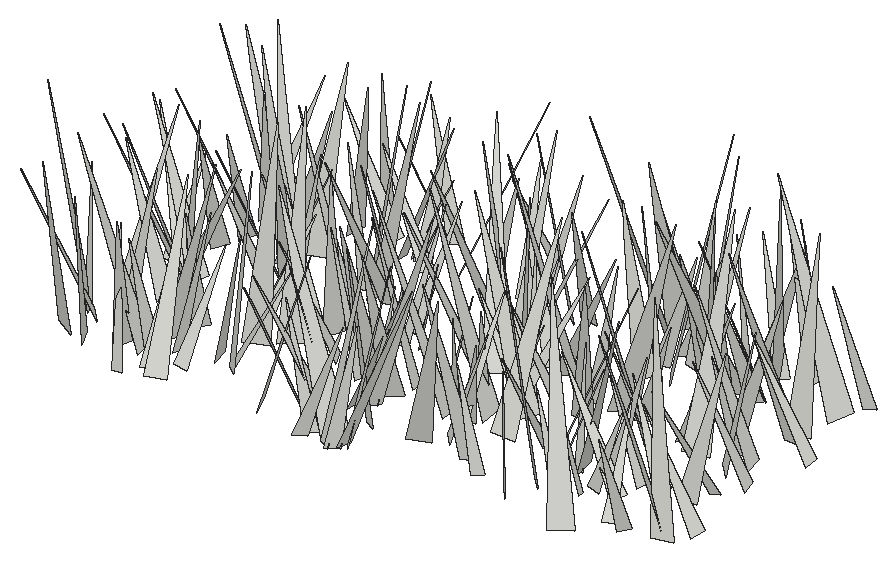
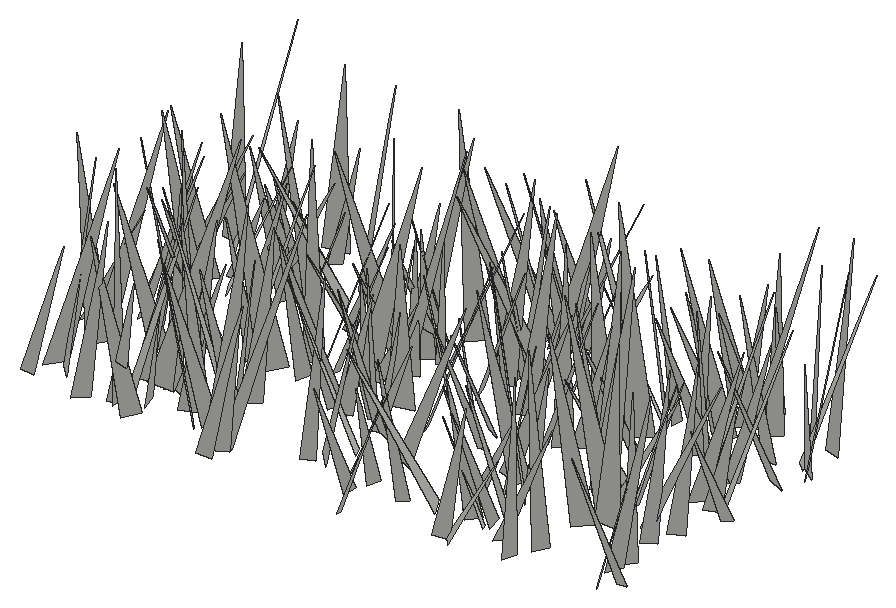
# SketchUp Ruby script. Lengths in inches.
U = 1.inch
M = Sketchup.active_model
def pt(a) = Geom::Point3d.new(a.map { |v| v * U })
def face(e, loops, mat)
  f = e.add_face(loops[0].map { |a| pt(a) })
  loops[1..].each { |l| e.add_face(l.map { |a| pt(a) }).erase! }
  f.material = f.back_material = mat if mat
  f
end
# faces: each face lists its corners as indices into pts; further lists are holes
def faces(e, pts, list, mat = nil) = list.each { |f| face(e, (f[0].is_a?(Array) ? f : [f]).map { |l| l.map { |i| pts[i] } }, mat) }
# xy, xz, yz: faces in a plane at the given z, y or x. An outline is a flat list of corners, or four numbers for a rectangle; further outlines are holes
def ring(l) = l.size == 4 ? [[l[0], l[1]], [l[2], l[1]], [l[2], l[3]], [l[0], l[3]]] : l.each_slice(2).to_a
def flat(e, list, mat, &to3) = list.each { |f| face(e, (f[0].is_a?(Array) ? f : [f]).map { |l| ring(l).map { |u, v| to3.(u, v) } }, mat) }
def xy(e, z, list, mat = nil) = flat(e, list, mat) { |x, y| [x, y, z] }
def xz(e, y, list, mat = nil) = flat(e, list, mat) { |x, z| [x, y, z] }
def yz(e, x, list, mat = nil) = flat(e, list, mat) { |y, z| [x, y, z] }
def lines(e, pts, list) = list.each { |a, b| e.add_line(pt(pts[a]), pt(pts[b])) }
# prism: a flat outline (further loops are holes) pulled along v
def prism(e, loops, v, mat = nil)
  f = face(e, loops, mat); d = Geom::Vector3d.new(v.map { |x| x * U })
  f.pushpull(f.normal.samedirection?(d) ? d.length : -d.length)
end
def box(e, o, s, mat = nil) = prism(e, [[o, [o[0] + s[0], o[1], o[2]], [o[0] + s[0], o[1] + s[1], o[2]], [o[0], o[1] + s[1], o[2]]]], [0, 0, s[2]], mat)
def at(x, y, z, deg = 0) = Geom::Transformation.translation(pt([x, y, z])) * Geom::Transformation.rotation(ORIGIN, Z_AXIS, deg.degrees)
def axes(o, x, y, z) = Geom::Transformation.new([*x, 0, *y, 0, *z, 0, *pt(o).to_a, 1])
def part(name) = M.definitions.add(name)
# library, detail: a bought-in or finely detailed component or shape, given as its bounding box
def library(name, o, s) = part(name).tap { |d| box(d.entities, o, s) }
def detail(e, o, s) = box(e.add_group.entities, o, s)
def put(e, d, t, mat = nil) = e.add_instance(d, t).tap { |i| i.material = mat if mat }
def group(e, t, mat = nil) = e.add_group.tap { |g| g.transformation = t; g.material = mat if mat }.entities
root = M.entities
c1 = part("fur_instance\#9")
p = [[0.8125,0,1.79],[0.67,-0.02,1.48],[0,-0.11,0],[0,0.11,0]]
faces(c1.entities,p,[[0,1,2,3]])
put(root,c1,axes([454.98,138.05,-21.66],[-2.48382,-6.27006,1.58629],[-6.2632,2.75568,1.08533],[1.61318,1.04494,6.65621]))
put(root,c1,axes([476.97,136.47,-21.66],[3.46953,-2.67132,1.40146],[-2.94376,-3.4648,0.68347],[-0.65905,1.41311,4.3251]))
put(root,c1,axes([474.43,136.51,-21.66],[3.70527,-2.55389,0.75103],[-2.66189,-3.54115,1.0909],[0.02774,1.32414,4.36593]))
put(root,c1,axes([456.74,137.75,-21.66],[4.97052,1.68586,2.30908],[2.28367,-5.12743,-1.17229],[-1.72012,-1.9358,5.11604]))
put(root,c1,axes([460.83,135.75,-21.66],[0.97276,4.45119,0.9772],[4.35496,-1.20232,1.14148],[-1.3425,-0.67498,4.41093]))
put(root,c1,axes([459.04,138.55,-21.66],[4.90376,-2.85552,0.72078],[-2.73926,-4.93651,-0.92072],[-1.08166,-0.44414,5.59939]))
put(root,c1,axes([475.1,138.93,-21.66],[-5.50457,-1.9976,0.13924],[-1.94432,5.42927,1.02602],[0.47897,-0.91798,5.76524]))
put(root,c1,axes([474.72,137.23,-21.66],[0.57769,-3.84784,2.16026],[-4.16363,-1.197,-1.01866],[-1.46176,1.88882,3.75525]))
put(root,c1,axes([461.22,138.875,-21.66],[3.60801,-2.69307,1.35493],[-2.4926,-3.85347,-1.02171],[-1.69571,-0.06573,4.3848]))
put(root,c1,axes([470.25,137.9,-21.66],[6.04949,2.12455,0.78775],[2.22415,-5.99674,-0.90711],[-0.43293,-1.1207,6.34722]))
put(root,c1,axes([455.41,140.42,-21.66],[-4.43936,-4.76816,0.23664],[-4.66276,4.39992,1.18262],[1.02469,-0.63608,6.40661]))
put(root,c1,axes([488.52,138.7,-21.66],[3.47548,2.68418,2.07766],[3.24177,-3.50628,-0.89294],[-1.00618,-2.02524,4.29959]))
put(root,c1,axes([460.34,139.04,-21.66],[-7.46338,-1.41905,1.28497],[-1.31215,7.55774,0.72509],[1.39396,-0.48353,7.56241]))
put(root,c1,axes([475.88,138.03,-21.66],[-6.89397,4.20656,1.53795],[4.42912,6.82252,1.19307],[0.66584,-1.82904,7.9874]))
put(root,c1,axes([477.26,137.21,-21.66],[6.02676,-0.13267,0.65935],[-0.25057,-5.95995,1.09109],[-0.62414,1.1116,5.92866]))
put(root,c1,axes([474.29,139.79,-21.66],[-3.67064,-4.64361,1.03864],[-4.58105,3.8034,0.81465],[1.28682,0.29416,5.86285]))
put(root,c1,axes([497.07,139.62,-21.66],[2.57242,-3.23839,0.522],[-3.12857,-2.6216,-0.84629],[-0.98573,-0.13048,4.04824]))
put(root,c1,axes([493.08,138.49,-21.66],[-3.28307,2.60382,1.30489],[2.8552,3.26547,0.66758],[0.57484,-1.34832,4.13676]))
put(root,c1,axes([462.01,137.22,-21.66],[-2.71251,3.20119,0.88639],[3.03008,2.85354,-1.03292],[1.36084,0.02704,4.06674]))
put(root,c1,axes([494.09,137.1875,-21.66],[-3.06885,7.2619,1.47031],[7.40414,2.94663,0.90053],[-0.27521,-1.70206,7.83212]))
put(root,c1,axes([480.46,140.51,-21.66],[3.94338,-5.9757,0.15667],[-5.94055,-3.89659,0.90015],[0.66588,0.62564,7.10275]))
put(root,c1,axes([463.16,136.61,-21.66],[-3.56616,5.34471,0.77163],[5.27091,3.64619,-0.89538],[1.17426,-0.13507,6.36253]))
put(root,c1,axes([472.08,139.48,-21.66],[-2.77092,-3.22119,0.17285],[-3.17409,2.68192,-0.90354],[-0.57541,0.71776,4.15182]))
put(root,c1,axes([476.3,136.5,-21.66],[3.93079,5.90323,1.06815],[5.73682,-4.07234,1.39466],[-1.7544,-0.09002,6.95371]))
put(root,c1,axes([477.33,137.4375,-21.66],[-3.93965,-2.75758,3.63418],[-3.8658,4.56754,-0.72493],[2.42222,2.80458,4.7539]))
put(root,c1,axes([498.85,141.17,-21.66],[-5.87389,-5.06073,1.31002],[-4.91563,6.01764,1.20596],[1.77871,-0.08191,7.65893]))
put(root,c1,axes([485.84,139.46,-21.66],[1.13242,-3.28388,1.61058],[-3.44754,-1.52145,-0.67814],[-1.2216,1.24962,3.40681]))
put(root,c1,axes([484.38,140.55,-21.66],[0.42808,-6.23217,1.75974],[-6.34467,-0.7568,-1.13683],[-1.29687,1.64535,6.14254]))
put(root,c1,axes([463.53,138.55,-21.66],[-0.65991,4.20046,0.70673],[4.09857,0.8209,-1.05196],[1.15975,-0.51096,4.1198]))
put(root,c1,axes([464.65,140.98,-21.66],[5.2345,0.58731,0.96902],[0.7581,-5.21929,-0.93179],[-0.84215,-1.04786,5.18428]))
put(root,c1,axes([476.94,140.09,-21.66],[-3.42512,-4.29344,1.99666],[-4.721,3.28594,-1.03273],[0.36395,2.21827,5.39431]))
put(root,c1,axes([462.21,140.04,-21.66],[4.7492,-0.22527,1.39473],[-0.44396,-4.88167,0.72329],[-1.34124,0.81823,4.6992]))
put(root,c1,axes([489.3,140.8125,-21.66],[-5.53788,-5.2946,2.37412],[-5.70348,5.57065,-0.88067],[1.06751,2.29618,7.61087]))
put(root,c1,axes([454.62,140.9,-21.66],[-6.58446,-3.61184,1.85584],[-3.84727,6.67992,-0.64953],[1.29924,1.4758,7.48189]))
put(root,c1,axes([499.61,140.12,-21.66],[-0.81741,7.52572,2.31704],[7.8363,0.54876,0.98214],[-0.77303,-2.39493,7.506]))
put(root,c1,axes([465.74,141.11,-21.66],[3.62695,2.69385,0.06353],[2.59465,-3.4627,-1.30122],[0.7271,-1.08099,4.32648]))
put(root,c1,axes([460.81,140.86,-21.66],[6.40804,-1.16691,1.44574],[-1.35043,-6.49108,0.74636],[-1.27601,1.00946,6.47052]))
put(root,c1,axes([457.27,141.23,-21.66],[1.6675,5.06938,1.93589],[5.41393,-1.41673,-0.95346],[0.36831,-2.12629,5.25072]))
put(root,c1,axes([495.77,139.76,-21.66],[-2.69846,2.82224,0.09608],[2.72603,2.63813,-0.93001],[0.73688,0.57546,3.79233]))
put(root,c1,axes([500.89,141.99,-21.66],[-4.33776,1.46199,0.55548],[1.55819,4.18055,1.16497],[0.13425,-1.28363,4.42678]))
put(root,c1,axes([466.2,140.21,-21.66],[3.82909,4.88275,1.88302],[4.81565,-4.20088,1.10051],[-2.04855,-0.74856,6.10673]))
put(root,c1,axes([475.77,143.82,-21.66],[3.11864,-5.68803,0.55795],[-5.6529,-3.16353,-0.65398],[-0.84244,0.17118,6.45383]))
put(root,c1,axes([454.52,140.9,-21.66],[1.72426,4.07776,1.35625],[4.04188,-2.03524,0.98061],[-1.4597,-0.81871,4.31736]))
put(root,c1,axes([492.26,141.43,-21.66],[-3.43885,-1.25141,0.28396],[-1.28081,3.29756,-0.97876],[-0.07859,1.01608,3.52615]))
put(root,c1,axes([481.72,141.8,-21.66],[3.27603,2.91205,0.73309],[2.99826,-3.11162,-1.03833],[0.1671,-1.26001,4.25844]))
put(root,c1,axes([461.38,143.34,-21.66],[3.51488,-3.51732,0.75482],[-3.443,-3.59499,-0.71937],[-1.04262,0.01399,4.9202]))
put(root,c1,axes([492.47,142.38,-21.66],[0.8957,-3.44027,0.95903],[-3.38159,-0.49886,1.36875],[1.14894,1.21373,3.28089]))
put(root,c1,axes([494.3,142.52,-21.66],[-4.30239,2.31555,0.00735],[2.25428,4.18495,1.12996],[-0.52922,-0.99839,4.75348]))
put(root,c1,axes([475.25,142.56,-21.66],[1.48907,3.83094,1.46531],[4.09712,-1.31638,-0.722],[0.19182,-1.62223,4.04625]))
put(root,c1,axes([475.52,142.05,-21.66],[6.84778,-1.68967,1.39359],[-1.92956,-6.81846,1.21431],[-1.03628,1.53061,6.94784]))
put(root,c1,axes([490.17,141.42,-21.66],[3.37937,2.22818,0.23171],[2.15143,-3.34494,0.78826],[-0.62436,0.53406,3.97033]))
put(root,c1,axes([490.44,144,-21.66],[6.84395,0.46131,0.76105],[0.6015,-6.74756,-1.31919],[-0.65589,-1.3745,6.73144]))
put(root,c1,axes([481.35,144.16,-21.66],[1.83451,-3.56347,0.05806],[-3.52397,-1.80394,0.62811],[0.53227,0.33851,3.95843]))
put(root,c1,axes([480.33,144.3,-21.66],[-0.97115,-4.17934,0.95629],[-4.09852,1.19278,1.05068],[1.25838,0.65947,4.16006]))
put(root,c1,axes([474.66,141.38,-21.66],[6.67299,1.88656,0.54903],[1.75109,-6.59185,1.3677],[-0.89119,1.17381,6.79833]))
put(root,c1,axes([487.18,144.6,-21.66],[-0.13278,-3.81265,0.23397],[-3.74221,0.08288,-0.77308],[-0.76609,0.25594,3.73581]))
put(root,c1,axes([465.32,143.67,-21.66],[-3.47226,6.33449,3.63746],[6.89094,4.17667,-0.69553],[2.42317,-2.80055,7.19017]))
put(root,c1,axes([492.625,143.8125,-21.66],[4.10289,-2.86128,0.97197],[-3.01034,-4.01302,0.89377],[-0.2636,1.29386,4.92156]))
put(root,c1,axes([472.33,145.94,-21.66],[3.11347,-5.57932,0.56956],[-5.54553,-3.1599,-0.63956],[-0.83685,0.18197,6.35716]))
put(root,c1,axes([470.2,145.46,-21.66],[-4.41173,-1.92667,0.46008],[-1.77307,4.34177,1.17998],[0.88316,-0.90777,4.66723]))
put(root,c1,axes([494.55,144.64,-21.66],[-3.60372,1.36671,1.25031],[1.68423,3.55609,0.96723],[0.77106,-1.37995,3.73084]))
put(root,c1,axes([458.37,146.03,-21.66],[-4.85913,-4.7221,0.69622],[-4.68141,4.90862,0.61965],[0.93132,0.03646,6.74725]))
put(root,c1,axes([496.72,143.75,-21.66],[-1.92431,3.57441,0.40694],[3.46774,1.72017,1.28872],[-0.95749,-0.95373,3.84949]))
put(root,c1,axes([479.86,144.0625,-21.66],[-7.1325,-1.97369,0.04131],[-1.9512,7.0246,-1.27181],[-0.29997,1.23662,7.29044]))
put(root,c1,axes([457.51,144.69,-21.66],[-4.78062,2.36193,1.12593],[2.54726,4.73726,0.87783],[0.59826,-1.2963,5.25951]))
put(root,c1,axes([490.34,143.66,-21.66],[1.055,3.81063,1.04337],[3.83467,-1.24762,0.6792],[-0.95124,-0.80317,3.89521]))
put(root,c1,axes([489.08,142.34,-21.66],[5.73522,3.47371,0.17785],[3.39582,-5.66618,1.16354],[-0.75282,0.90483,6.60345]))
put(root,c1,axes([481.44,143.03,-21.66],[-0.33332,4.6985,0.41104],[4.65173,0.39553,-0.74898],[0.77866,-0.35159,4.65038]))
put(root,c1,axes([496.18,145.11,-21.66],[-4.80301,-2.64529,0.12183],[-2.62964,4.73476,-0.865],[-0.31202,0.81591,5.41463]))
put(root,c1,axes([481.99,145.61,-21.66],[-7.83608,-0.63477,1.59162],[-0.4911,7.96997,0.76075],[1.64165,-0.64574,7.82485]))
put(root,c1,axes([497.83,144.72,-21.66],[-1.7832,4.7887,2.83203],[5.02838,2.65983,-1.33139],[2.38064,-2.03113,4.93345]))
put(root,c1,axes([472.91,144.23,-21.66],[-4.76571,-0.2474,0.30777],[-0.30187,4.68534,-0.90794],[0.25457,0.92426,4.68496]))
put(root,c1,axes([498.58,146.54,-21.66],[-0.19761,-4.29399,0.26182],[-4.09062,0.10641,-1.34218],[-1.33181,0.31028,4.08362]))
put(root,c1,axes([480.77,146.41,-21.66],[0.8236,-4.35079,0.44599],[-4.32851,-0.74586,0.71716],[0.62636,0.56649,4.3696]))
put(root,c1,axes([473.95,145.6875,-21.66],[-0.58036,-3.55618,1.37675],[-3.59236,0.97706,1.00942],[1.27936,1.13031,3.45894]))
put(root,c1,axes([457.67,145.51,-21.66],[5.28703,-2.12696,0.17156],[-2.11759,-5.17319,1.12251],[0.26309,1.10465,5.58719]))
put(root,c1,axes([455.2,143.16,-21.66],[2.05142,5.93925,0.09208],[5.90467,-2.04959,0.65232],[-0.64654,0.12643,6.2496]))
put(root,c1,axes([484.12,144.02,-21.66],[-1.25446,7.26591,1.58891],[7.27727,1.53186,-1.25954],[1.53602,-1.32352,7.26503]))
put(root,c1,axes([476.24,145.5625,-21.66],[-5.31837,-1.43549,0.4315],[-1.49067,5.23198,-0.96754],[0.15722,1.04767,5.42306]))
put(root,c1,axes([483.2,144.99,-21.66],[3.56009,0.21869,0.65734],[0.01468,-3.46445,1.07311],[-0.69261,1.05069,3.40155]))
put(root,c1,axes([455.43,148.24,-21.66],[-4.61159,-4.4726,0.38091],[-4.39573,4.61032,0.9157],[0.90928,-0.396,6.35865]))
put(root,c1,axes([466.86,145.05,-21.66],[-5.99811,4.4385,2.51735],[4.45899,6.44808,-0.74453],[2.48087,-0.8583,7.4245]))
put(root,c1,axes([468.24,147.54,-21.66],[5.51508,-3.1001,1.56666],[-3.03836,-5.73026,-0.64316],[-1.68328,0.18611,6.29389]))
put(root,c1,axes([477.88,146.55,-21.66],[3.15545,2.01724,0.79775],[2.15051,-3.09372,-0.68323],[-0.2846,-1.01105,3.6823]))
put(root,c1,axes([464.3,145.4,-21.66],[0.4921,4.23207,0.57816],[4.10963,-0.31046,-1.22532],[1.16432,-0.69285,4.08059]))
put(root,c1,axes([483.78,146.88,-21.66],[-6.02527,4.37662,1.94606],[4.73834,5.90349,1.39383],[0.70004,-2.28907,7.31546]))
put(root,c1,axes([486.54,148.76,-21.66],[1.84605,-6.6162,0.27609],[-6.51912,-1.76548,1.28157],[1.16252,0.60597,6.74831]))
put(root,c1,axes([456.93,147.38,-21.66],[3.49606,4.56093,2.47636],[5.16488,-3.35013,-1.12142],[-0.50841,-2.67048,5.63622]))
put(root,c1,axes([467.35,146.99,-21.66],[-4.02277,2.62654,1.01722],[2.78428,3.97624,0.74391],[0.42575,-1.18612,4.74637]))
put(root,c1,axes([499.65,148.47,-21.66],[-4.7933,-0.97536,0.74224],[-0.77682,4.73507,1.20565],[0.94805,-1.05153,4.74061]))
put(root,c1,axes([484.64,148.93,-21.66],[-4.25051,-1.02119,0.70994],[-0.79222,4.17184,1.25768],[0.95876,-1.08007,4.18663]))
put(root,c1,axes([462.7,150.39,-21.66],[5.93446,-4.51627,0.11992],[-4.41947,-5.84426,-1.3935],[-0.93776,-1.03771,7.32616]))
put(root,c1,axes([457.64,147.7,-21.66],[-5.5849,2.54638,0.93821],[2.66389,5.55377,0.78405],[0.51763,-1.10771,6.08773]))
put(root,c1,axes([482.02,148.29,-21.66],[-2.52559,2.65872,0.46687],[2.62617,2.27215,1.26725],[-0.62447,-1.19747,3.44114]))
put(root,c1,axes([491.17,149.02,-21.66],[-5.74367,-4.09689,1.01684],[-4.21686,5.6466,-1.0688],[0.19121,1.46278,6.97366]))
put(root,c1,axes([464.03,148.77,-21.66],[-1.49797,-4.88201,2.75569],[-5.27998,2.18724,1.00478],[1.88406,2.24805,5.00683]))
put(root,c1,axes([497.22,149.12,-21.66],[4.01593,3.70117,1.52807],[3.99587,-3.8439,-1.19115],[-0.25835,-1.92018,5.32987]))
put(root,c1,axes([482.36,147.59,-21.66],[1.65691,4.63189,0.02775],[4.518,-1.60961,-1.09423],[1.0212,-0.39403,4.79608]))
put(root,c1,axes([476.14,150.81,-21.66],[-5.06216,-2.56794,0.53616],[-2.44101,5.03776,1.08155],[0.96086,-0.73072,5.57226]))
put(root,c1,axes([473.18,149.72,-21.66],[3.34183,1.38887,0.77255],[1.56239,-3.2005,-1.00466],[-0.29109,-1.23347,3.4767]))
put(root,c1,axes([456.21,148.1,-21.66],[-3.43494,4.07646,0.13435],[4.04677,3.38429,0.77755],[-0.50915,-0.60283,5.27368]))
put(root,c1,axes([460.22,150.58,-21.66],[-4.26767,-0.91045,0.71231],[-0.70932,4.21373,1.13607],[0.91278,-0.98229,4.21323]))
put(root,c1,axes([468.82,148.84,-21.66],[-7.05105,-1.29004,0.36767],[-1.33665,6.92247,-1.34515],[0.11284,1.38992,7.04075]))
put(root,c1,axes([496.81,151.07,-21.66],[3.89618,-1.88557,1.1779],[-1.51971,-3.99347,-1.36592],[-1.62275,-0.78732,4.1073]))
put(root,c1,axes([454.74,148.46,-21.66],[-0.81178,3.59213,0.55552],[3.51446,0.92094,-0.81938],[0.92765,-0.34562,3.5904]))
put(root,c1,axes([498.1875,150.71,-21.66],[-6.30832,-1.1114,1.05664],[-1.00602,6.37534,0.69964],[1.15742,-0.51611,6.36715]))
put(root,c1,axes([456.05,151.74,-21.66],[3.84252,-3.67557,0.42443],[-3.56655,-3.84235,-0.9854],[-0.98471,-0.42605,5.2253]))
put(root,c1,axes([482.69,148.37,-21.66],[-4.63028,1.37895,0.71291],[1.15549,4.55932,-1.31404],[1.03661,1.07721,4.64912]))
put(root,c1,axes([461.4,150.82,-21.66],[-3.04212,-3.44962,0.11938],[-3.35963,2.92271,-1.15727],[-0.79185,0.85236,4.45141]))
put(root,c1,axes([489.52,150.86,-21.66],[3.13596,-3.23192,0.2957],[-3.22644,-3.06024,0.76944],[0.35051,0.74607,4.43707]))
put(root,c1,axes([462.7,150.54,-21.66],[1.59006,-7.38899,3.46765],[-7.94346,-2.21328,-1.07372],[-1.87702,3.10714,7.48148]))
put(root,c1,axes([487.81,151.04,-21.66],[6.25642,-5.32962,1.03257],[-5.42827,-6.12142,1.29455],[0.06986,1.65444,8.11614]))
put(root,c1,axes([462.29,148.79,-21.66],[4.05537,2.07279,0.17475],[1.9711,-3.95155,1.12829],[-0.66463,0.92835,4.41242]))
put(root,c1,axes([472.55,148.89,-21.66],[1.79845,4.31058,0.12569],[4.2592,-1.79684,0.67963],[-0.67534,0.14702,4.621]))
put(root,c1,axes([468.5,152.53,-21.66],[-0.3519,-5.66898,0.64957],[-5.59847,0.21723,-1.13712],[-1.1029,0.70611,5.5649]))
put(root,c1,axes([484.61,150.93,-21.66],[-7.32124,-3.15954,0.71739],[-3.23761,7.2018,-1.32279],[0.12329,1.49974,7.86343]))
put(root,c1,axes([485.79,150.64,-21.66],[4.38322,-1.64948,1.59394],[-1.93146,-4.50849,0.64578],[-1.2373,1.19448,4.63858]))
put(root,c1,axes([494.61,149.63,-21.66],[-2.78975,7.45432,2.27613],[7.61508,3.12201,-0.8911],[1.66081,-1.79348,7.90921]))
put(root,c1,axes([492.91,150.43,-21.66],[5.00649,-0.69371,1.01239],[-0.92226,-4.93206,1.18126],[-0.80969,1.32843,4.91435]))
put(root,c1,axes([456.72,153.59,-21.66],[4.17409,-3.35782,0.27535],[-3.2273,-4.11088,-1.20788],[-0.96712,-0.77425,5.2191]))
put(root,c1,axes([457.68,152.86,-21.66],[-3.27123,-4.88451,0.3113],[-4.82797,3.15879,-1.17003],[-0.80376,0.90546,5.76111]))
put(root,c1,axes([460.55,152.63,-21.66],[5.42547,-4.53511,0.52895],[-4.56014,-5.3411,0.98008],[0.2284,1.09004,7.00303]))
put(root,c1,axes([471.8,150.76,-21.66],[0.88242,4.55252,0.64978],[4.54635,-0.76413,-0.82042],[0.6916,-0.78549,4.5641]))
put(root,c1,axes([480.07,150.99,-21.66],[-4.86729,-1.78674,2.25978],[-2.35287,5.02555,-1.09424],[1.66225,1.88173,5.06809]))
put(root,c1,axes([479.28,151.99,-21.66],[0.33455,3.97904,1.71347],[4.11253,0.24873,-1.38056],[1.36232,-1.72801,3.74683]))
put(root,c1,axes([482.08,152.18,-21.66],[4.93305,-2.19664,0.15391],[-2.18894,-4.85066,0.92924],[0.23965,0.9109,5.31946]))
put(root,c1,axes([478.96,151.72,-21.66],[-6.73527,-1.87686,1.53677],[-2.12146,6.75676,-1.04577],[1.17629,1.43931,6.91323]))
put(root,c1,axes([498.45,154.38,-21.66],[-0.93689,-7.58778,0.99671],[-7.63501,0.85799,-0.64504],[-0.52389,1.06539,7.61814]))
put(root,c1,axes([478.85,149.92,-21.66],[-3.36629,7.35026,0.38103],[7.33966,3.3212,0.77612],[-0.54849,-0.66835,8.0471]))
put(root,c1,axes([500.75,153.14,-21.66],[-4.62797,0.36048,0.06702],[0.36662,4.56134,0.78248],[0.00509,-0.78533,4.57556]))
put(root,c1,axes([492.17,153.64,-21.66],[7.07527,1.73735,2.55738],[2.12787,-7.36989,-0.88027],[-2.24293,-1.5114,7.23207]))
put(root,c1,axes([481.05,152.68,-21.66],[-3.33055,3.67395,0.98734],[3.8043,3.21801,0.85849],[0.0046,-1.30837,4.884]))
put(root,c1,axes([467.34,154.36,-21.66],[3.26712,2.26093,2.86418],[3.20778,-3.61207,-0.80776],[-1.73938,-2.41465,3.89016]))
put(root,c1,axes([478.22,153.11,-21.66],[-2.47066,2.78913,0.64805],[2.82871,2.24449,1.12431],[-0.44456,-1.21919,3.55237]))
put(root,c1,axes([466.3,152.96,-21.66],[-0.19493,4.51759,1.73565],[4.75586,-0.14282,0.90585],[-0.89608,-1.74071,4.43013]))
put(root,c1,axes([494.83,153.35,-21.66],[4.67154,-2.82363,0.84685],[-2.94301,-4.55853,1.0353],[-0.16964,1.32674,5.35951]))
put(root,c1,axes([467.43,152.7,-21.66],[6.54484,-1.1484,2.12677],[-1.53141,-6.71985,1.08414],[-1.86996,1.48383,6.55579]))
put(root,c1,axes([491.85,156.96,-21.66],[1.8393,-7.94223,0.20343],[-7.82957,-1.84746,-1.33722],[-1.34842,-0.10629,8.04201]))
put(root,c1,axes([465.96,154.0625,-21.66],[6.04593,4.4435,2.18806],[4.86244,-5.98205,-1.28733],[-0.94282,-2.35709,7.39194]))
put(root,c1,axes([474.54,155.1,-21.66],[-1.00098,-5.50903,0.83943],[-5.47181,0.81017,-1.20786],[-1.05515,1.02481,5.46739]))
put(root,c1,axes([492.6,151.46,-21.66],[3.19327,6.60837,0.52108],[6.51338,-3.23542,1.11669],[-1.23207,0.02336,7.254]))
put(root,c1,axes([460.02,153.48,-21.66],[-1.69454,7.12423,1.83382],[7.32335,1.45532,1.11334],[-0.69716,-2.02889,7.23786]))
put(root,c1,axes([491.04,156.72,-21.66],[0.94954,-6.1364,0.24208],[-6.03443,-0.88683,1.18943],[1.14,0.41683,6.09444]))
put(root,c1,axes([486.33,155.07,-21.66],[-4.53938,3.59005,2.40826],[4.08452,4.7056,0.68422],[1.41595,-2.06469,5.74685]))
put(root,c1,axes([461.17,154.35,-21.66],[-3.27295,5.40819,2.7555],[5.57889,3.91368,-1.05481],[2.39109,-1.7286,6.23283]))
put(root,c1,axes([456.03,156.32,-21.66],[5.00192,-1.81934,1.03799],[-1.65,-5.07776,-0.94895],[-1.29032,-0.55947,5.23724]))
put(root,c1,axes([493.34,156.91,-21.66],[2.17041,-4.52553,0.56409],[-4.42394,-2.24099,-0.95709],[-1.10786,0.0828,4.92697]))
put(root,c1,axes([498.17,155.03,-21.66],[4.86014,-4.74094,2.82615],[-5.30574,-5.05065,0.65171],[-1.52079,2.46963,6.75816]))
put(root,c1,axes([457.46,155.75,-21.66],[-5.88104,-3.53705,0.94417],[-3.64814,5.81133,-0.9531],[0.30541,1.30636,6.79625]))
put(root,c1,axes([493.27,157.81,-21.66],[-4.06699,-5.2197,0.56162],[-5.13541,4.10303,0.94539],[1.09007,-0.14467,6.54919]))
put(root,c1,axes([487.39,155.1,-21.66],[-5.21816,-1.76906,1.50642],[-2.07355,5.2165,-1.05669],[1.04846,1.51216,5.4076]))
put(root,c1,axes([477.78,153.125,-21.66],[1.53889,6.65129,0.3221],[6.53467,-1.57198,1.24039],[-1.28121,-0.02868,6.71336]))
put(root,c1,axes([488.67,158.25,-21.66],[4.29462,-4.11505,0.26594],[-3.98176,-4.23808,-1.27765],[-1.07236,-0.74374,5.80905]))
put(root,c1,axes([477.53,155.81,-21.66],[5.0651,3.0377,0.15182],[3.00547,-4.95362,-1.15532],[0.46672,-1.0677,5.79207]))
put(root,c1,axes([490.27,156.95,-21.66],[-1.57238,-4.56901,1.11948],[-4.65933,1.35009,-1.0341],[-0.64787,1.37945,4.72005]))
put(root,c1,axes([479.28,158.4375,-21.66],[-0.0268,-5.65268,0.22398],[-5.53849,0.07185,1.15049],[1.15241,0.21383,5.53443]))
put(root,c1,axes([486.15,156.86,-21.66],[3.07396,-3.53335,0.83024],[-3.61315,-2.87553,1.13994],[0.34489,1.36741,4.5425]))
put(root,c1,axes([456.26,157.49,-21.66],[-6.02827,1.48886,1.73676],[1.72693,6.17226,0.7029],[1.50026,-1.12234,6.1695]))
put(root,c1,axes([461.34,158.29,-21.66],[5.97247,-1.71505,1.0533],[-1.60325,-6.04797,-0.7569],[-1.21673,-0.44932,6.16757]))
put(root,c1,axes([467.66,157.26,-21.66],[-3.1989,2.68909,0.37978],[2.66785,3.00183,1.21655],[-0.50792,-1.16886,3.99802]))
put(root,c1,axes([487.98,157.74,-21.66],[-0.07815,-6.05054,2.52953],[-6.4447,0.53908,1.09033],[1.2138,2.47266,5.952]))
put(root,c1,axes([487.625,155.89,-21.66],[6.38887,5.18246,1.59043],[5.07791,-6.58181,1.04866],[-1.89794,-0.16426,8.1594]))
put(root,c1,axes([497.56,159.09,-21.66],[4.54557,4.08977,3.87164],[5.12111,-5.0718,-0.65499],[-2.34307,-3.15097,6.07942]))
put(root,c1,axes([478.53,157.75,-21.66],[2.96491,4.33641,3.25393],[4.46173,-4.05854,1.34327],[-3.07985,-1.70497,5.07846]))
put(root,c1,axes([484.5,159.67,-21.66],[-4.58981,-6.81856,1.14154],[-6.9132,4.53833,-0.68805],[0.05895,1.33156,8.19058]))
put(root,c1,axes([465.78,158.23,-21.66],[3.19259,1.80159,0.09548],[1.75198,-3.04965,-1.03811],[0.43061,-0.9494,3.51578]))
put(root,c1,axes([498.67,158.61,-21.66],[-7.81883,2.51294,1.68172],[2.76611,7.82758,1.16397],[1.22135,-1.64052,8.12983]))
put(root,c1,axes([471.63,158.78,-21.66],[1.56073,-4.1385,0.9971],[-4.17951,-1.28812,1.1957],[0.80812,1.33073,4.25833]))
put(root,c1,axes([465.54,157.54,-21.66],[4.89085,0.64493,0.58721],[0.56841,-4.89366,0.64042],[-0.66156,0.56328,4.89144]))
put(root,c1,axes([466.84,157.875,-21.66],[-2.42701,4.03219,1.90827],[4.11447,2.86278,-0.81615],[1.72373,-1.15601,4.63496]))
put(root,c1,axes([484.32,161.03,-21.66],[5.05065,-5.78899,0.88016],[-5.66798,-5.12516,-1.18448],[-1.47008,-0.1285,7.59069]))
put(root,c1,axes([486.57,158.7,-21.66],[4.08139,-3.20586,0.61223],[-3.2526,-3.91407,1.18774],[0.27008,1.30866,5.05219]))
put(root,c1,axes([455.82,159.67,-21.66],[-3.08221,-2.2445,0.63722],[-2.14243,3.14072,0.69983],[0.92405,-0.20483,3.74807]))
put(root,c1,axes([463.95,158.92,-21.66],[-4.51711,1.79985,0.33219],[1.82954,4.41557,0.95372],[-0.05124,-1.00862,4.76803]))
put(root,c1,axes([464.62,157.09,-21.66],[4.77639,3.07128,1.21309],[2.81816,-4.90311,1.31748],[-1.72115,0.49496,5.52367]))
put(root,c1,axes([492.72,159.91,-21.66],[7.08469,1.17747,2.52447],[1.61288,-7.35894,-1.094],[-2.27113,-1.55299,7.09806]))
put(root,c1,axes([475.82,158.89,-21.66],[-4.15206,-1.52587,0.16301],[-1.50616,3.96212,-1.27574],[-0.29385,1.25209,4.2356]))
put(root,c1,axes([462.26,160.2,-21.66],[5.48977,-0.87036,1.92832],[-0.64898,-5.79667,-0.76876],[-2.01365,-0.50463,5.50492]))
put(root,c1,axes([454.75,158.65,-21.66],[1.35315,4.35582,0.79538],[4.34518,-1.14634,-1.11449],[0.85157,-1.07217,4.42291]))
put(root,c1,axes([474.34,158.19,-21.66],[-3.56654,2.39752,0.7344],[2.22273,3.6139,-1.00345],[1.16058,0.44646,4.17868]))
put(root,c1,axes([499.32,160.54,-21.66],[0.38107,-4.3176,1.24457],[-4.35966,-0.65774,-0.94692],[-1.08815,1.12319,4.22969]))
put(root,c1,axes([491.2,158.9,-21.66],[-4.4304,-0.23548,0.66281],[-0.42328,4.26855,-1.31284],[0.56178,1.35914,4.23796]))
put(root,c1,axes([469.55,158.09,-21.66],[5.6659,3.07924,0.02777],[3.03508,-5.59401,1.03936],[-0.52039,0.90013,6.36426]))
put(root,c1,axes([491.08,160.76,-21.66],[4.31446,-3.71791,0.40504],[-3.72385,-4.21342,0.9907],[0.3462,1.01276,5.60856]))
put(root,c1,axes([487.67,159.07,-21.66],[-4.49953,-3.59508,3.80394],[-4.60675,5.10137,-0.62788],[2.48443,2.94818,5.72505]))
put(root,c1,axes([494.8125,161,-21.66],[4.62611,-3.05223,2.53258],[-2.97331,-5.24406,-0.88892],[-2.62479,0.5609,5.47054]))
put(root,c1,axes([492.79,160.17,-21.66],[1.4221,-3.78822,2.5832],[-4.25079,-2.10312,-0.74405],[-1.71882,2.06693,3.97736]))
put(root,c1,axes([466.5,160.89,-21.66],[-2.71564,-2.49022,0.0198],[-2.39499,2.6036,-1.03032],[-0.68234,0.77224,3.53756]))
put(root,c1,axes([473.71,162.37,-21.66],[-3.49973,-1.74713,0.54329],[-1.50598,3.41664,1.28623],[1.03907,-0.93268,3.69408]))
put(root,c1,axes([474.87,159.87,-21.66],[3.51726,-1.23078,1.44078],[-1.67757,-3.4351,1.16087],[-0.88116,1.62697,3.54095]))
put(root,c1,axes([467.04,160.86,-21.66],[1.69917,-3.99461,2.49122],[-4.30676,-2.38859,-0.89256],[-1.90128,1.84064,4.24822]))
put(root,c1,axes([484.5,161.97,-21.66],[0.91416,-4.94391,1.27953],[-4.9749,-1.15567,-0.91103],[-1.1532,1.06645,4.94449]))
